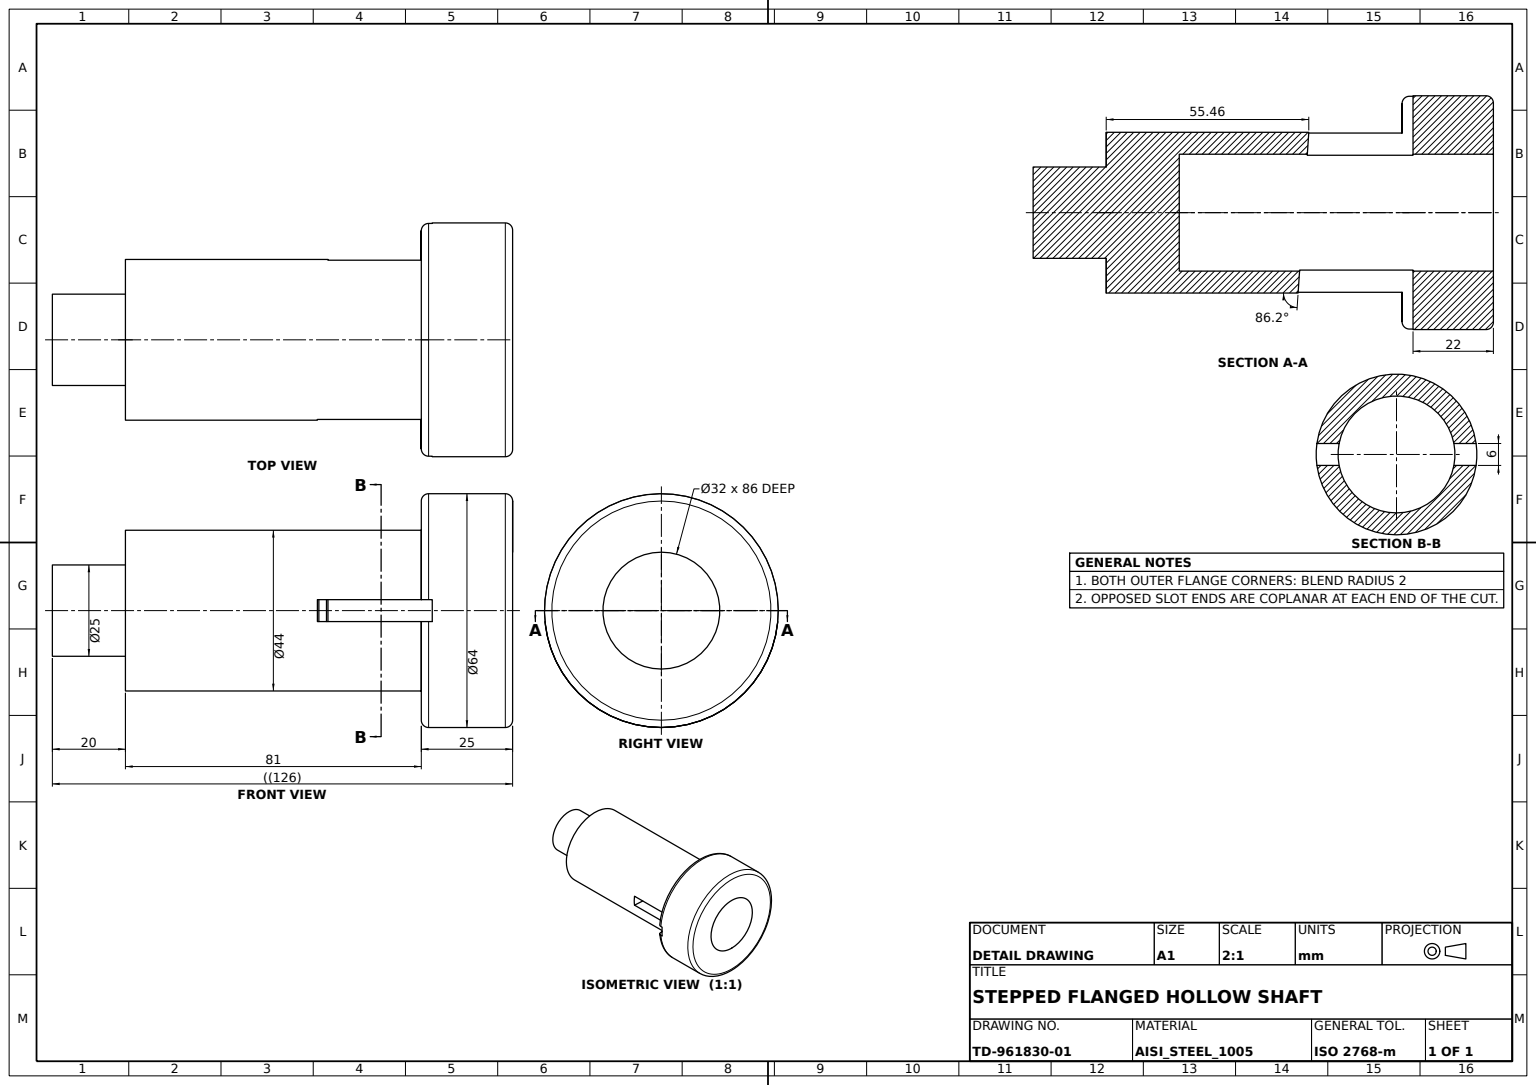
ISO-10303-21;
HEADER;
FILE_DESCRIPTION((''),'2;1');
FILE_NAME('','',(''),(''),'','','');
FILE_SCHEMA(('AUTOMOTIVE_DESIGN'));
ENDSEC;
DATA;
#1=APPLICATION_CONTEXT('');
#2=PRODUCT_CONTEXT('',#1,'mechanical');
#3=PRODUCT('','','',(#2));
#4=PRODUCT_DEFINITION_FORMATION('','',#3);
#5=PRODUCT_DEFINITION_CONTEXT('',#1,'design');
#6=PRODUCT_DEFINITION('','',#4,#5);
#7=PRODUCT_DEFINITION_SHAPE('','',#6);
#8=(LENGTH_UNIT()NAMED_UNIT(*)SI_UNIT(.MILLI.,.METRE.));
#9=(NAMED_UNIT(*)PLANE_ANGLE_UNIT()SI_UNIT($,.RADIAN.));
#10=(NAMED_UNIT(*)SI_UNIT($,.STERADIAN.)SOLID_ANGLE_UNIT());
#11=UNCERTAINTY_MEASURE_WITH_UNIT(LENGTH_MEASURE(0.005),#8,'distance_accuracy_value','');
#12=(GEOMETRIC_REPRESENTATION_CONTEXT(3)GLOBAL_UNCERTAINTY_ASSIGNED_CONTEXT((#11))GLOBAL_UNIT_ASSIGNED_CONTEXT((#8,#9,#10))REPRESENTATION_CONTEXT('',''));
#13=CARTESIAN_POINT('',(-3.,-31.859065,3.));
#14=VERTEX_POINT('',#13);
#15=CARTESIAN_POINT('',(-3.,-15.716234,3.));
#16=VERTEX_POINT('',#15);
#17=CARTESIAN_POINT('',(-3.,78.812304,3.));
#18=DIRECTION('',(0.,-1.,0.));
#19=VECTOR('',#18,1000.);
#20=LINE('',#17,#19);
#21=EDGE_CURVE('',#14,#16,#20,.F.);
#22=ORIENTED_EDGE('',*,*,#21,.F.);
#23=CARTESIAN_POINT('',(-3.,-31.859065,2.));
#24=VERTEX_POINT('',#23);
#25=CARTESIAN_POINT('',(-3.,-31.859065,25.));
#26=DIRECTION('',(0.,0.,-1.));
#27=VECTOR('',#26,1000.);
#28=LINE('',#25,#27);
#29=EDGE_CURVE('',#14,#24,#28,.T.);
#30=ORIENTED_EDGE('',*,*,#29,.T.);
#31=CARTESIAN_POINT('',(-3.,-29.849623,0.));
#32=VERTEX_POINT('',#31);
#33=CARTESIAN_POINT('',(-3.,-31.859065,1.470511));
#34=CARTESIAN_POINT('',(-3.,-31.419758,0.433866));
#35=CARTESIAN_POINT('',(-3.,-30.379042,0.));
#36=B_SPLINE_CURVE_WITH_KNOTS('',3,(#23,#33,#34,#35,#31),.UNSPECIFIED.,.F.,.F.,(4,1,4),(0.,0.001565884,0.003131767),.UNSPECIFIED.);
#37=EDGE_CURVE('',#24,#32,#36,.T.);
#38=ORIENTED_EDGE('',*,*,#37,.T.);
#39=CARTESIAN_POINT('',(-3.,-21.794495,0.));
#40=VERTEX_POINT('',#39);
#41=CARTESIAN_POINT('',(-3.,0.,0.));
#42=DIRECTION('',(0.,1.,0.));
#43=VECTOR('',#42,1000.);
#44=LINE('',#41,#43);
#45=EDGE_CURVE('',#32,#40,#44,.T.);
#46=ORIENTED_EDGE('',*,*,#45,.T.);
#47=CARTESIAN_POINT('',(-3.,-21.794495,-28.447589));
#48=VERTEX_POINT('',#47);
#49=CARTESIAN_POINT('',(-3.,-21.794495,-81.));
#50=DIRECTION('',(0.,0.,1.));
#51=VECTOR('',#50,1000.);
#52=LINE('',#49,#51);
#53=EDGE_CURVE('',#40,#48,#52,.F.);
#54=ORIENTED_EDGE('',*,*,#53,.T.);
#55=CARTESIAN_POINT('',(-3.,-15.716234,-28.043871));
#56=VERTEX_POINT('',#55);
#57=CARTESIAN_POINT('',(-3.,-77.418488,-32.14213));
#58=DIRECTION('',(0.,0.997801468,0.0662739));
#59=VECTOR('',#58,1000.);
#60=LINE('',#57,#59);
#61=EDGE_CURVE('',#56,#48,#60,.F.);
#62=ORIENTED_EDGE('',*,*,#61,.F.);
#63=CARTESIAN_POINT('',(-3.,-15.716234,-61.));
#64=LINE('',#63,#51);
#65=EDGE_CURVE('',#56,#16,#64,.T.);
#66=ORIENTED_EDGE('',*,*,#65,.T.);
#67=EDGE_LOOP('',(#22,#30,#38,#46,#54,#62,#66));
#68=FACE_BOUND('',#67,.T.);
#69=DIRECTION('',(1.,0.,0.));
#70=AXIS2_PLACEMENT_3D('',#41,#69,#26);
#71=PLANE('',#70);
#72=ADVANCED_FACE('',(#68),#71,.T.);
#73=CARTESIAN_POINT('',(3.,-15.716234,-28.043871));
#74=VERTEX_POINT('',#73);
#75=CARTESIAN_POINT('',(0.,0.,-27.));
#76=DIRECTION('',(0.,-0.0662739,0.997801468));
#77=AXIS2_PLACEMENT_3D('',#75,#76,#58);
#78=ELLIPSE('',#77,16.035254,16.);
#79=EDGE_CURVE('',#74,#56,#78,.F.);
#80=ORIENTED_EDGE('',*,*,#79,.T.);
#81=ORIENTED_EDGE('',*,*,#61,.T.);
#82=CARTESIAN_POINT('',(3.,-21.794495,-28.447589));
#83=VERTEX_POINT('',#82);
#84=ELLIPSE('',#77,22.048474,22.);
#85=EDGE_CURVE('',#48,#83,#84,.T.);
#86=ORIENTED_EDGE('',*,*,#85,.T.);
#87=CARTESIAN_POINT('',(3.,-77.418488,-32.14213));
#88=LINE('',#87,#59);
#89=EDGE_CURVE('',#74,#83,#88,.F.);
#90=ORIENTED_EDGE('',*,*,#89,.F.);
#91=EDGE_LOOP('',(#80,#81,#86,#90));
#92=FACE_BOUND('',#91,.T.);
#93=DIRECTION('',(0.,-0.997801468,-0.0662739));
#94=AXIS2_PLACEMENT_3D('',#87,#76,#93);
#95=PLANE('',#94);
#96=ADVANCED_FACE('',(#92),#95,.T.);
#97=CARTESIAN_POINT('',(12.5,0.,-101.));
#98=VERTEX_POINT('',#97);
#99=CARTESIAN_POINT('',(0.,0.,-101.));
#100=AXIS2_PLACEMENT_3D('',#99,#26,#69);
#101=CIRCLE('',#100,12.5);
#102=EDGE_CURVE('',#98,#98,#101,.T.);
#103=ORIENTED_EDGE('',*,*,#102,.T.);
#104=EDGE_LOOP('',(#103));
#105=FACE_BOUND('',#104,.T.);
#106=DIRECTION('',(-1.,0.,0.));
#107=AXIS2_PLACEMENT_3D('',#99,#26,#106);
#108=PLANE('',#107);
#109=ADVANCED_FACE('',(#105),#108,.T.);
#110=CARTESIAN_POINT('',(3.,15.716234,3.));
#111=VERTEX_POINT('',#110);
#112=CARTESIAN_POINT('',(-3.,15.716234,3.));
#113=VERTEX_POINT('',#112);
#114=CARTESIAN_POINT('',(0.,0.,3.));
#115=AXIS2_PLACEMENT_3D('',#114,#26,#42);
#116=CIRCLE('',#115,16.);
#117=EDGE_CURVE('',#111,#113,#116,.F.);
#118=ORIENTED_EDGE('',*,*,#117,.T.);
#119=CARTESIAN_POINT('',(-3.,31.859065,3.));
#120=VERTEX_POINT('',#119);
#121=EDGE_CURVE('',#113,#120,#20,.F.);
#122=ORIENTED_EDGE('',*,*,#121,.T.);
#123=CARTESIAN_POINT('',(3.,31.859065,3.));
#124=VERTEX_POINT('',#123);
#125=CIRCLE('',#115,32.);
#126=EDGE_CURVE('',#120,#124,#125,.T.);
#127=ORIENTED_EDGE('',*,*,#126,.T.);
#128=CARTESIAN_POINT('',(3.,78.812304,3.));
#129=LINE('',#128,#19);
#130=EDGE_CURVE('',#111,#124,#129,.F.);
#131=ORIENTED_EDGE('',*,*,#130,.F.);
#132=EDGE_LOOP('',(#118,#122,#127,#131));
#133=FACE_BOUND('',#132,.T.);
#134=AXIS2_PLACEMENT_3D('',#128,#26,#42);
#135=PLANE('',#134);
#136=ADVANCED_FACE('',(#133),#135,.T.);
#137=ORIENTED_EDGE('',*,*,#37,.F.);
#138=CARTESIAN_POINT('',(-3.,31.859065,2.));
#139=VERTEX_POINT('',#138);
#140=CARTESIAN_POINT('',(0.,0.,2.));
#141=AXIS2_PLACEMENT_3D('',#140,#50,#69);
#142=CIRCLE('',#141,32.);
#143=EDGE_CURVE('',#139,#24,#142,.T.);
#144=ORIENTED_EDGE('',*,*,#143,.F.);
#145=CARTESIAN_POINT('',(-3.,29.849623,0.));
#146=VERTEX_POINT('',#145);
#147=CARTESIAN_POINT('',(-3.,30.379083,0.));
#148=CARTESIAN_POINT('',(-3.,31.417696,0.43186));
#149=CARTESIAN_POINT('',(-3.,31.859065,1.470467));
#150=B_SPLINE_CURVE_WITH_KNOTS('',3,(#145,#147,#148,#149,#138),.UNSPECIFIED.,.F.,.F.,(4,1,4),(0.,0.00156589,0.003131779),.UNSPECIFIED.);
#151=EDGE_CURVE('',#146,#139,#150,.T.);
#152=ORIENTED_EDGE('',*,*,#151,.F.);
#153=CARTESIAN_POINT('',(0.,0.,0.));
#154=AXIS2_PLACEMENT_3D('',#153,#50,#69);
#155=CIRCLE('',#154,30.);
#156=EDGE_CURVE('',#32,#146,#155,.F.);
#157=ORIENTED_EDGE('',*,*,#156,.F.);
#158=EDGE_LOOP('',(#137,#144,#152,#157));
#159=FACE_BOUND('',#158,.T.);
#160=TOROIDAL_SURFACE('',#141,30.,2.);
#161=ADVANCED_FACE('',(#159),#160,.T.);
#162=ORIENTED_EDGE('',*,*,#65,.F.);
#163=ORIENTED_EDGE('',*,*,#79,.F.);
#164=CARTESIAN_POINT('',(3.,-15.716234,3.));
#165=VERTEX_POINT('',#164);
#166=CARTESIAN_POINT('',(3.,-15.716234,-61.));
#167=LINE('',#166,#51);
#168=EDGE_CURVE('',#74,#165,#167,.T.);
#169=ORIENTED_EDGE('',*,*,#168,.T.);
#170=EDGE_CURVE('',#16,#165,#116,.F.);
#171=ORIENTED_EDGE('',*,*,#170,.F.);
#172=EDGE_LOOP('',(#162,#163,#169,#171));
#173=FACE_BOUND('',#172,.T.);
#174=CARTESIAN_POINT('',(-3.,15.716234,-25.956129));
#175=VERTEX_POINT('',#174);
#176=CARTESIAN_POINT('',(-3.,15.716234,-61.));
#177=LINE('',#176,#51);
#178=EDGE_CURVE('',#113,#175,#177,.F.);
#179=ORIENTED_EDGE('',*,*,#178,.F.);
#180=ORIENTED_EDGE('',*,*,#117,.F.);
#181=CARTESIAN_POINT('',(3.,15.716234,-25.956129));
#182=VERTEX_POINT('',#181);
#183=CARTESIAN_POINT('',(3.,15.716234,-61.));
#184=LINE('',#183,#51);
#185=EDGE_CURVE('',#111,#182,#184,.F.);
#186=ORIENTED_EDGE('',*,*,#185,.T.);
#187=EDGE_CURVE('',#175,#182,#78,.F.);
#188=ORIENTED_EDGE('',*,*,#187,.F.);
#189=EDGE_LOOP('',(#179,#180,#186,#188));
#190=FACE_BOUND('',#189,.T.);
#191=CARTESIAN_POINT('',(16.,0.,25.));
#192=VERTEX_POINT('',#191);
#193=CARTESIAN_POINT('',(0.,0.,25.));
#194=AXIS2_PLACEMENT_3D('',#193,#50,#69);
#195=CIRCLE('',#194,16.);
#196=EDGE_CURVE('',#192,#192,#195,.T.);
#197=ORIENTED_EDGE('',*,*,#196,.T.);
#198=EDGE_LOOP('',(#197));
#199=FACE_BOUND('',#198,.T.);
#200=CARTESIAN_POINT('',(16.,0.,-61.));
#201=VERTEX_POINT('',#200);
#202=CARTESIAN_POINT('',(0.,0.,-61.));
#203=AXIS2_PLACEMENT_3D('',#202,#50,#69);
#204=CIRCLE('',#203,16.);
#205=EDGE_CURVE('',#201,#201,#204,.F.);
#206=ORIENTED_EDGE('',*,*,#205,.T.);
#207=EDGE_LOOP('',(#206));
#208=FACE_BOUND('',#207,.T.);
#209=CYLINDRICAL_SURFACE('',#203,16.);
#210=ADVANCED_FACE('',(#173,#190,#199,#208),#209,.F.);
#211=ORIENTED_EDGE('',*,*,#196,.F.);
#212=EDGE_LOOP('',(#211));
#213=FACE_BOUND('',#212,.T.);
#214=CARTESIAN_POINT('',(30.,0.,25.));
#215=VERTEX_POINT('',#214);
#216=CIRCLE('',#194,30.);
#217=EDGE_CURVE('',#215,#215,#216,.T.);
#218=ORIENTED_EDGE('',*,*,#217,.T.);
#219=EDGE_LOOP('',(#218));
#220=FACE_BOUND('',#219,.T.);
#221=PLANE('',#194);
#222=ADVANCED_FACE('',(#213,#220),#221,.T.);
#223=CARTESIAN_POINT('',(-3.,21.794495,0.));
#224=VERTEX_POINT('',#223);
#225=EDGE_CURVE('',#224,#146,#44,.T.);
#226=ORIENTED_EDGE('',*,*,#225,.F.);
#227=AXIS2_PLACEMENT_3D('',#153,#26,#69);
#228=CIRCLE('',#227,22.);
#229=EDGE_CURVE('',#40,#224,#228,.T.);
#230=ORIENTED_EDGE('',*,*,#229,.F.);
#231=ORIENTED_EDGE('',*,*,#45,.F.);
#232=ORIENTED_EDGE('',*,*,#156,.T.);
#233=EDGE_LOOP('',(#226,#230,#231,#232));
#234=FACE_BOUND('',#233,.T.);
#235=PLANE('',#154);
#236=ADVANCED_FACE('',(#234),#235,.F.);
#237=ORIENTED_EDGE('',*,*,#102,.F.);
#238=EDGE_LOOP('',(#237));
#239=FACE_BOUND('',#238,.T.);
#240=CARTESIAN_POINT('',(12.5,0.,-81.));
#241=VERTEX_POINT('',#240);
#242=CARTESIAN_POINT('',(0.,0.,-81.));
#243=AXIS2_PLACEMENT_3D('',#242,#26,#69);
#244=CIRCLE('',#243,12.5);
#245=EDGE_CURVE('',#241,#241,#244,.T.);
#246=ORIENTED_EDGE('',*,*,#245,.T.);
#247=EDGE_LOOP('',(#246));
#248=FACE_BOUND('',#247,.T.);
#249=AXIS2_PLACEMENT_3D('',#99,#50,#69);
#250=CYLINDRICAL_SURFACE('',#249,12.5);
#251=ADVANCED_FACE('',(#239,#248),#250,.T.);
#252=ORIENTED_EDGE('',*,*,#178,.T.);
#253=CARTESIAN_POINT('',(-3.,21.794495,-25.552411));
#254=VERTEX_POINT('',#253);
#255=EDGE_CURVE('',#254,#175,#60,.F.);
#256=ORIENTED_EDGE('',*,*,#255,.F.);
#257=CARTESIAN_POINT('',(-3.,21.794495,-81.));
#258=LINE('',#257,#51);
#259=EDGE_CURVE('',#254,#224,#258,.T.);
#260=ORIENTED_EDGE('',*,*,#259,.T.);
#261=ORIENTED_EDGE('',*,*,#225,.T.);
#262=ORIENTED_EDGE('',*,*,#151,.T.);
#263=CARTESIAN_POINT('',(-3.,31.859065,25.));
#264=LINE('',#263,#27);
#265=EDGE_CURVE('',#139,#120,#264,.F.);
#266=ORIENTED_EDGE('',*,*,#265,.T.);
#267=ORIENTED_EDGE('',*,*,#121,.F.);
#268=EDGE_LOOP('',(#252,#256,#260,#261,#262,#266,#267));
#269=FACE_BOUND('',#268,.T.);
#270=ADVANCED_FACE('',(#269),#71,.T.);
#271=CARTESIAN_POINT('',(3.,-29.849623,0.));
#272=VERTEX_POINT('',#271);
#273=CARTESIAN_POINT('',(3.,-21.794495,0.));
#274=VERTEX_POINT('',#273);
#275=CARTESIAN_POINT('',(3.,0.,0.));
#276=LINE('',#275,#43);
#277=EDGE_CURVE('',#272,#274,#276,.T.);
#278=ORIENTED_EDGE('',*,*,#277,.T.);
#279=CARTESIAN_POINT('',(3.,21.794495,0.));
#280=VERTEX_POINT('',#279);
#281=EDGE_CURVE('',#280,#274,#228,.T.);
#282=ORIENTED_EDGE('',*,*,#281,.F.);
#283=CARTESIAN_POINT('',(3.,29.849623,0.));
#284=VERTEX_POINT('',#283);
#285=EDGE_CURVE('',#280,#284,#276,.T.);
#286=ORIENTED_EDGE('',*,*,#285,.T.);
#287=EDGE_CURVE('',#284,#272,#155,.F.);
#288=ORIENTED_EDGE('',*,*,#287,.T.);
#289=EDGE_LOOP('',(#278,#282,#286,#288));
#290=FACE_BOUND('',#289,.T.);
#291=ADVANCED_FACE('',(#290),#235,.F.);
#292=ORIENTED_EDGE('',*,*,#130,.T.);
#293=CARTESIAN_POINT('',(3.,31.859065,2.));
#294=VERTEX_POINT('',#293);
#295=CARTESIAN_POINT('',(3.,31.859065,25.));
#296=LINE('',#295,#27);
#297=EDGE_CURVE('',#294,#124,#296,.F.);
#298=ORIENTED_EDGE('',*,*,#297,.F.);
#299=CARTESIAN_POINT('',(3.,31.859065,1.470511));
#300=CARTESIAN_POINT('',(3.,31.419758,0.433866));
#301=CARTESIAN_POINT('',(3.,30.379042,0.));
#302=B_SPLINE_CURVE_WITH_KNOTS('',3,(#293,#299,#300,#301,#283),.UNSPECIFIED.,.F.,.F.,(4,1,4),(0.,0.001565884,0.003131767),.UNSPECIFIED.);
#303=EDGE_CURVE('',#294,#284,#302,.T.);
#304=ORIENTED_EDGE('',*,*,#303,.T.);
#305=ORIENTED_EDGE('',*,*,#285,.F.);
#306=CARTESIAN_POINT('',(3.,21.794495,-25.552411));
#307=VERTEX_POINT('',#306);
#308=CARTESIAN_POINT('',(3.,21.794495,-81.));
#309=LINE('',#308,#51);
#310=EDGE_CURVE('',#307,#280,#309,.T.);
#311=ORIENTED_EDGE('',*,*,#310,.F.);
#312=EDGE_CURVE('',#307,#182,#88,.F.);
#313=ORIENTED_EDGE('',*,*,#312,.T.);
#314=ORIENTED_EDGE('',*,*,#185,.F.);
#315=EDGE_LOOP('',(#292,#298,#304,#305,#311,#313,#314));
#316=FACE_BOUND('',#315,.T.);
#317=AXIS2_PLACEMENT_3D('',#275,#69,#26);
#318=PLANE('',#317);
#319=ADVANCED_FACE('',(#316),#318,.F.);
#320=ORIENTED_EDGE('',*,*,#217,.F.);
#321=EDGE_LOOP('',(#320));
#322=FACE_BOUND('',#321,.T.);
#323=CARTESIAN_POINT('',(32.,0.,23.));
#324=VERTEX_POINT('',#323);
#325=CARTESIAN_POINT('',(0.,0.,23.));
#326=AXIS2_PLACEMENT_3D('',#325,#50,#69);
#327=CIRCLE('',#326,32.);
#328=EDGE_CURVE('',#324,#324,#327,.F.);
#329=ORIENTED_EDGE('',*,*,#328,.F.);
#330=EDGE_LOOP('',(#329));
#331=FACE_BOUND('',#330,.T.);
#332=TOROIDAL_SURFACE('',#326,30.,2.);
#333=ADVANCED_FACE('',(#322,#331),#332,.T.);
#334=ORIENTED_EDGE('',*,*,#205,.F.);
#335=EDGE_LOOP('',(#334));
#336=FACE_BOUND('',#335,.T.);
#337=PLANE('',#203);
#338=ADVANCED_FACE('',(#336),#337,.T.);
#339=CARTESIAN_POINT('',(3.,-31.859065,3.));
#340=VERTEX_POINT('',#339);
#341=EDGE_CURVE('',#340,#165,#129,.F.);
#342=ORIENTED_EDGE('',*,*,#341,.F.);
#343=EDGE_CURVE('',#340,#14,#125,.T.);
#344=ORIENTED_EDGE('',*,*,#343,.T.);
#345=ORIENTED_EDGE('',*,*,#21,.T.);
#346=ORIENTED_EDGE('',*,*,#170,.T.);
#347=EDGE_LOOP('',(#342,#344,#345,#346));
#348=FACE_BOUND('',#347,.T.);
#349=ADVANCED_FACE('',(#348),#135,.T.);
#350=ORIENTED_EDGE('',*,*,#312,.F.);
#351=EDGE_CURVE('',#307,#254,#84,.T.);
#352=ORIENTED_EDGE('',*,*,#351,.T.);
#353=ORIENTED_EDGE('',*,*,#255,.T.);
#354=ORIENTED_EDGE('',*,*,#187,.T.);
#355=EDGE_LOOP('',(#350,#352,#353,#354));
#356=FACE_BOUND('',#355,.T.);
#357=ADVANCED_FACE('',(#356),#95,.T.);
#358=ORIENTED_EDGE('',*,*,#29,.F.);
#359=ORIENTED_EDGE('',*,*,#343,.F.);
#360=CARTESIAN_POINT('',(3.,-31.859065,2.));
#361=VERTEX_POINT('',#360);
#362=CARTESIAN_POINT('',(3.,-31.859065,25.));
#363=LINE('',#362,#27);
#364=EDGE_CURVE('',#340,#361,#363,.T.);
#365=ORIENTED_EDGE('',*,*,#364,.T.);
#366=EDGE_CURVE('',#361,#294,#142,.T.);
#367=ORIENTED_EDGE('',*,*,#366,.T.);
#368=ORIENTED_EDGE('',*,*,#297,.T.);
#369=ORIENTED_EDGE('',*,*,#126,.F.);
#370=ORIENTED_EDGE('',*,*,#265,.F.);
#371=ORIENTED_EDGE('',*,*,#143,.T.);
#372=EDGE_LOOP('',(#358,#359,#365,#367,#368,#369,#370,#371));
#373=FACE_BOUND('',#372,.T.);
#374=ORIENTED_EDGE('',*,*,#328,.T.);
#375=EDGE_LOOP('',(#374));
#376=FACE_BOUND('',#375,.T.);
#377=AXIS2_PLACEMENT_3D('',#193,#26,#106);
#378=CYLINDRICAL_SURFACE('',#377,32.);
#379=ADVANCED_FACE('',(#373,#376),#378,.T.);
#380=CARTESIAN_POINT('',(3.,-30.379083,0.));
#381=CARTESIAN_POINT('',(3.,-31.417696,0.43186));
#382=CARTESIAN_POINT('',(3.,-31.859065,1.470467));
#383=B_SPLINE_CURVE_WITH_KNOTS('',3,(#271,#380,#381,#382,#360),.UNSPECIFIED.,.F.,.F.,(4,1,4),(0.,0.00156589,0.003131779),.UNSPECIFIED.);
#384=EDGE_CURVE('',#272,#361,#383,.T.);
#385=ORIENTED_EDGE('',*,*,#384,.F.);
#386=ORIENTED_EDGE('',*,*,#287,.F.);
#387=ORIENTED_EDGE('',*,*,#303,.F.);
#388=ORIENTED_EDGE('',*,*,#366,.F.);
#389=EDGE_LOOP('',(#385,#386,#387,#388));
#390=FACE_BOUND('',#389,.T.);
#391=ADVANCED_FACE('',(#390),#160,.T.);
#392=CARTESIAN_POINT('',(3.,-21.794495,-81.));
#393=LINE('',#392,#51);
#394=EDGE_CURVE('',#274,#83,#393,.F.);
#395=ORIENTED_EDGE('',*,*,#394,.T.);
#396=ORIENTED_EDGE('',*,*,#85,.F.);
#397=ORIENTED_EDGE('',*,*,#53,.F.);
#398=ORIENTED_EDGE('',*,*,#229,.T.);
#399=ORIENTED_EDGE('',*,*,#259,.F.);
#400=ORIENTED_EDGE('',*,*,#351,.F.);
#401=ORIENTED_EDGE('',*,*,#310,.T.);
#402=ORIENTED_EDGE('',*,*,#281,.T.);
#403=EDGE_LOOP('',(#395,#396,#397,#398,#399,#400,#401,#402));
#404=FACE_BOUND('',#403,.T.);
#405=CARTESIAN_POINT('',(22.,0.,-81.));
#406=VERTEX_POINT('',#405);
#407=CIRCLE('',#243,22.);
#408=EDGE_CURVE('',#406,#406,#407,.T.);
#409=ORIENTED_EDGE('',*,*,#408,.F.);
#410=EDGE_LOOP('',(#409));
#411=FACE_BOUND('',#410,.T.);
#412=AXIS2_PLACEMENT_3D('',#242,#50,#69);
#413=CYLINDRICAL_SURFACE('',#412,22.);
#414=ADVANCED_FACE('',(#404,#411),#413,.T.);
#415=ORIENTED_EDGE('',*,*,#384,.T.);
#416=ORIENTED_EDGE('',*,*,#364,.F.);
#417=ORIENTED_EDGE('',*,*,#341,.T.);
#418=ORIENTED_EDGE('',*,*,#168,.F.);
#419=ORIENTED_EDGE('',*,*,#89,.T.);
#420=ORIENTED_EDGE('',*,*,#394,.F.);
#421=ORIENTED_EDGE('',*,*,#277,.F.);
#422=EDGE_LOOP('',(#415,#416,#417,#418,#419,#420,#421));
#423=FACE_BOUND('',#422,.T.);
#424=ADVANCED_FACE('',(#423),#318,.F.);
#425=ORIENTED_EDGE('',*,*,#408,.T.);
#426=EDGE_LOOP('',(#425));
#427=FACE_BOUND('',#426,.T.);
#428=ORIENTED_EDGE('',*,*,#245,.F.);
#429=EDGE_LOOP('',(#428));
#430=FACE_BOUND('',#429,.T.);
#431=AXIS2_PLACEMENT_3D('',#242,#26,#106);
#432=PLANE('',#431);
#433=ADVANCED_FACE('',(#427,#430),#432,.T.);
#434=CLOSED_SHELL('',(#72,#96,#109,#136,#161,#210,#222,#236,#251,#270,#291,#319,#333,#338,#349,#357,#379,#391,#414,#424,#433));
#435=MANIFOLD_SOLID_BREP('',#434);
#436=ADVANCED_BREP_SHAPE_REPRESENTATION('',(#435),#12);
#437=SHAPE_DEFINITION_REPRESENTATION(#7,#436);
ENDSEC;
END-ISO-10303-21;
